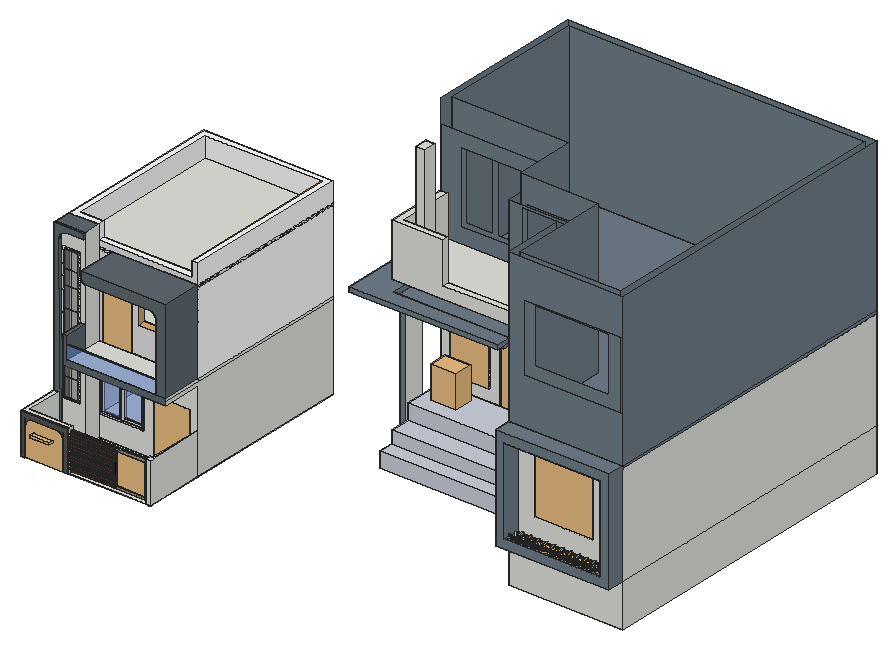
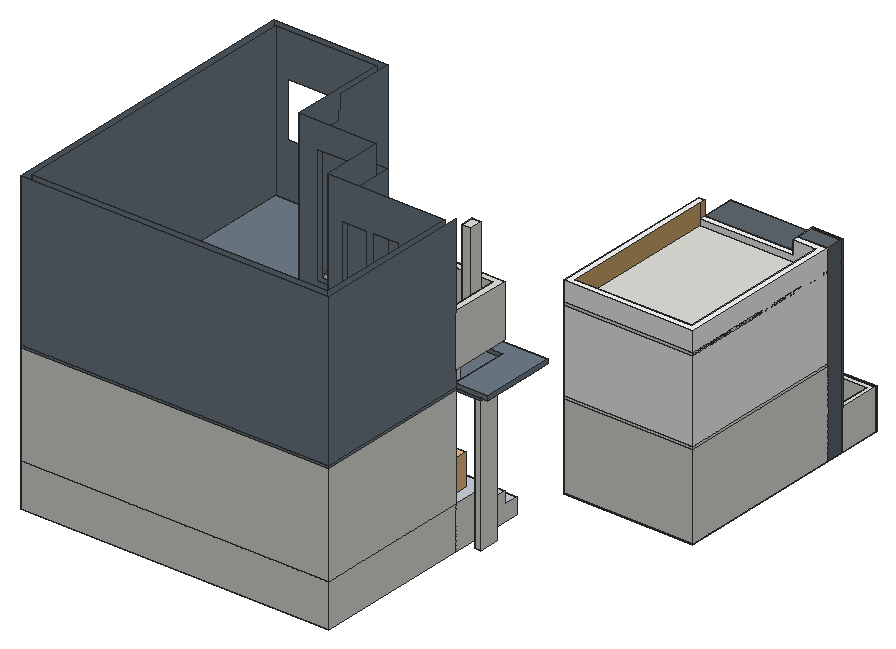
# SketchUp Ruby script. Lengths in inches.
U = 1.inch
M = Sketchup.active_model
def pt(a) = Geom::Point3d.new(a.map { |v| v * U })
def face(e, loops, mat)
  f = e.add_face(loops[0].map { |a| pt(a) })
  loops[1..].each { |l| e.add_face(l.map { |a| pt(a) }).erase! }
  f.material = f.back_material = mat if mat
  f
end
# faces: each face lists its corners as indices into pts; further lists are holes
def faces(e, pts, list, mat = nil) = list.each { |f| face(e, (f[0].is_a?(Array) ? f : [f]).map { |l| l.map { |i| pts[i] } }, mat) }
# xy, xz, yz: faces in a plane at the given z, y or x. An outline is a flat list of corners, or four numbers for a rectangle; further outlines are holes
def ring(l) = l.size == 4 ? [[l[0], l[1]], [l[2], l[1]], [l[2], l[3]], [l[0], l[3]]] : l.each_slice(2).to_a
def flat(e, list, mat, &to3) = list.each { |f| face(e, (f[0].is_a?(Array) ? f : [f]).map { |l| ring(l).map { |u, v| to3.(u, v) } }, mat) }
def xy(e, z, list, mat = nil) = flat(e, list, mat) { |x, y| [x, y, z] }
def xz(e, y, list, mat = nil) = flat(e, list, mat) { |x, z| [x, y, z] }
def yz(e, x, list, mat = nil) = flat(e, list, mat) { |y, z| [x, y, z] }
def lines(e, pts, list) = list.each { |a, b| e.add_line(pt(pts[a]), pt(pts[b])) }
# prism: a flat outline (further loops are holes) pulled along v
def prism(e, loops, v, mat = nil)
  f = face(e, loops, mat); d = Geom::Vector3d.new(v.map { |x| x * U })
  f.pushpull(f.normal.samedirection?(d) ? d.length : -d.length)
end
def box(e, o, s, mat = nil) = prism(e, [[o, [o[0] + s[0], o[1], o[2]], [o[0] + s[0], o[1] + s[1], o[2]], [o[0], o[1] + s[1], o[2]]]], [0, 0, s[2]], mat)
def at(x, y, z, deg = 0) = Geom::Transformation.translation(pt([x, y, z])) * Geom::Transformation.rotation(ORIGIN, Z_AXIS, deg.degrees)
def axes(o, x, y, z) = Geom::Transformation.new([*x, 0, *y, 0, *z, 0, *pt(o).to_a, 1])
def part(name) = M.definitions.add(name)
# library, detail: a bought-in or finely detailed component or shape, given as its bounding box
def library(name, o, s) = part(name).tap { |d| box(d.entities, o, s) }
def detail(e, o, s) = box(e.add_group.entities, o, s)
def put(e, d, t, mat = nil) = e.add_instance(d, t).tap { |i| i.material = mat if mat }
def group(e, t, mat = nil) = e.add_group.tap { |g| g.transformation = t; g.material = mat if mat }.entities
root = M.entities
M.materials.add("Aluminum_Bumpy_5cm\#1").color = [83, 85, 85]
M.materials.add("Heather_Brim").color = [96, 66, 40]
M.materials.add("Heather_Brim1").color = [73, 50, 31]
M.materials.add("Heather_Cuffs").color = [111, 126, 137]
M.materials.add("Heather_Hat").color = [155, 148, 119]
M.materials.add("Lily_Blonde").color = [204, 166, 109]
M.materials.add("Lily_Light").color = [247, 247, 197]
M.materials.add("[Color E05]").color = [255, 255, 0]
M.materials.add("[Color M01]").color = [226, 226, 226]
M.materials.add("[Color M02]").color = [198, 198, 198]
M.materials.add("[Color M09]").color = [0, 0, 0]
M.materials.add("[Formica Speckled Grey]").color = [94, 105, 111]
M.materials.add("[Marble Carrara Floor Tile]").color = [204, 208, 219]
M.materials.add("[Quartz Light Grey]").color = [251, 251, 252]
M.materials.add("[Translucent Glass Blue]").color = [100, 149, 237]
M.materials["[Translucent Glass Blue]"].alpha = 0.5
M.materials.add("[Translucent Glass Gray]").color = [128, 128, 128]
M.materials["[Translucent Glass Gray]"].alpha = 0.5
M.materials.add("[Wood Veneer 01]").color = [120, 70, 37]
c1 = library("Plant",[0,0,0],[12.59,12.59,14.16])
c2 = library("Door+01",[0,-2.84,-4],[33.31,7.1,94])
c3 = library("BANK+STOEL+MET+RONDE+LEUNING",[-13.09,-13.32,0],[26.18,25.9,25.63])
c4 = library("Group\#16",[13.45,-2,0],[53.92,2,50.83])
c5 = part("Horizontal slat")
xy(c5.entities,0,[[0,0,63.76,1]])
xy(c5.entities,1.75,[[0,0,63.76,1]],"Heather_Brim")
xz(c5.entities,0,[[0,0,63.76,1.75]],"Heather_Brim")
xz(c5.entities,1,[[0,0,63.76,1.75]])
yz(c5.entities,0,[[0,0,1,1.75]])
yz(c5.entities,63.76,[[0,0,1,1.75]])
c6 = part("Group\#20")
put(c6.entities,c5,at(0,-1,0))
c7 = library("Group\#19",[0,-1,-41.22],[40.08,1.95,42.17])
c8 = part("Difference\#2")
xy(c8.entities,0,[[0,-85,0,-27,6.6875,-27,6.6875,-77.875,63.37,-77.875,63.37,-85],[63.37,-85,67.37,-77.875],[177.37,-85,177.37,-77.875,181.37,-77.875,181.37,0,184,0,184,-85],[0,0,0,240,184,240,184,0,171.48,0,171.48,9,175,9,175,231,9,231,9,9,120.45,9,120.45,0]])
xy(c8.entities,2.75,[[131.125,-83.25,131.125,-82.25,67.37,-82.25,67.37,-80.625,177.37,-80.625,177.37,-83.25]])
xy(c8.entities,5.83,[[134.21,-83.25,174.29,-82.25]])
xy(c8.entities,29.83,[[42.47,0,105.68,9]])
xy(c8.entities,51.72,[[134.21,-83.25,174.29,-82.25]])
xy(c8.entities,54.8,[[131.125,-83.25,177.37,-83.25,177.37,-80.625,67.37,-80.625,67.37,-82.25,131.125,-82.25]])
xy(c8.entities,57.55,[[0,-85,63.37,-85,63.37,-77.875,6.6875,-77.875,6.6875,-27,0,-27],[63.37,-85,67.37,-77.875],[177.37,-85,184,-85,184,0,181.37,0,181.37,-77.875,177.37,-77.875]])
xy(c8.entities,79.83,[[42.47,0,105.68,9]])
xy(c8.entities,81,[[120.45,0,171.48,9]])
xy(c8.entities,115.1,[[36.47,-57,36.47,-24,42.47,-24,42.47,0,184,0,184,-57]],"[Formica Speckled Grey]")
xy(c8.entities,124,[[42.47,-57,168.74,0],[168.74,-57,171.48,0],[171.48,-57,184,0]])
xy(c8.entities,155,[[36.47,-57,42.47,-24]],"[Formica Speckled Grey]")
xy(c8.entities,228.74,[[69.63,-57,159.02,0]],"[Formica Speckled Grey]")
xy(c8.entities,244,[[62,-57,184,0]],"[Formica Speckled Grey]")
xz(c8.entities,-85,[[0,0,67.37,57.55],[177.37,0,184,57.55]])
xz(c8.entities,-83.25,[[[131.125,2.75,177.37,54.8],[134.21,5.83,174.29,51.72]]],"Heather_Hat")
xz(c8.entities,-82.25,[[67.37,2.75,131.125,53.05]])
xz(c8.entities,-82.25,[[134.21,5.83,174.29,48.6875],[134.21,49.64,174.29,51.72]],"Heather_Hat")
xz(c8.entities,-80.625,[[67.37,2.75,177.37,54.8]])
xz(c8.entities,-77.875,[[6.6875,0,63.37,57.55],[63.37,0,67.37,57.55],[177.37,0,181.37,57.55]])
xz(c8.entities,-57,[[36.47,115.1,184,115.1,184,124,42.47,124,42.47,155,36.47,155],[168.74,124,184,124,184,244,62,244,62,236.37,62.07,235.37,62.26,234.39,62.58,233.45,63.02,232.55,63.58,231.72,64.24,230.97,64.99,230.3125,65.82,229.76,66.71,229.32,67.66,229,68.64,228.8,69.63,228.74,159.02,228.74,160.29,228.65,161.54,228.41,162.74,228,163.88,227.4375,164.9375,226.73,165.89,225.89,166.73,224.9375,167.4375,223.88,168,222.74,168.41,221.54,168.65,220.29,168.74,219.02]],"[Formica Speckled Grey]")
xz(c8.entities,-27,[[0,0,6.6875,57.55]])
xz(c8.entities,-24,[[36.47,115.1,42.47,155]])
xz(c8.entities,0,[[0,0,42.47,120],[42.47,0,120.45,0,120.45,81,171.48,81,171.48,0,181.37,0,181.37,57.55,184,57.55,184,115.1,42.47,115.1,42.47,79.83,105.68,79.83,105.68,29.83,42.47,29.83],[181.37,0,184,57.55],[168.74,124,168.74,219.02,168.65,220.29,168.41,221.54,168,222.74,167.4375,223.88,166.73,224.9375,165.89,225.89,164.9375,226.73,163.88,227.4375,162.74,228,161.54,228.41,160.29,228.65,159.02,228.74,69.63,228.74,68.64,228.8,67.66,229,66.71,229.32,65.82,229.76,64.99,230.3125,64.24,230.97,63.58,231.72,63.02,232.55,62.58,233.45,62.26,234.39,62.07,235.37,62,236.37,62,244,184,244,184,124]])
xz(c8.entities,9,[[[9,0,9,120,175,120,175,0,171.48,0,171.48,81,120.45,81,120.45,0],[42.47,29.83,105.68,79.83]]])
xz(c8.entities,231,[[9,0,175,120]])
xz(c8.entities,240,[[0,0,184,120]])
yz(c8.entities,0,[[-85,0,-27,57.55],[0,0,240,120]])
yz(c8.entities,6.6875,[[-77.875,0,-27,57.55]])
yz(c8.entities,9,[[9,0,231,120]])
yz(c8.entities,36.47,[[-57,115.1,-24,155]],"[Formica Speckled Grey]")
yz(c8.entities,42.47,[[0,29.83,9,79.83],[-24,115.1,0,124]])
yz(c8.entities,42.47,[[-57,124,-24,155]],"[Formica Speckled Grey]")
yz(c8.entities,62,[[-57,236.37,0,244]],"[Formica Speckled Grey]")
yz(c8.entities,67.37,[[[-85,0,-77.875,57.55],[-82.25,2.75,-80.625,54.8]],[-82.25,2.75,-80.625,54.8]])
yz(c8.entities,105.68,[[0,29.83,9,79.83]])
yz(c8.entities,120.45,[[0,0,9,81]])
yz(c8.entities,131.125,[[-83.25,2.75,-82.25,53.05],[-83.25,53.05,-82.25,54.8]])
yz(c8.entities,134.21,[[-83.25,5.83,-82.25,51.72]])
yz(c8.entities,168.74,[[-57,124,0,219.02]],"[Formica Speckled Grey]")
yz(c8.entities,171.48,[[0,0,9,81]])
yz(c8.entities,174.29,[[-83.25,5.83,-82.25,51.72]])
yz(c8.entities,175,[[9,0,231,120]])
yz(c8.entities,177.37,[[[-85,0,-77.875,57.55],[-83.25,2.75,-80.625,54.8]]])
yz(c8.entities,181.37,[[-77.875,0,0,57.55]])
yz(c8.entities,184,[[-85,0,0,57.55],[0,0,240,0,240,120,-57,120,-57,115.1,0,115.1],[-57,120,0,124]])
yz(c8.entities,184,[[-57,124,0,244]],"[Formica Speckled Grey]")
p = [[168.74,-57,219.02],[168.65,-57,220.29],[168.65,0,220.29],[168.74,0,219.02],[168.41,-57,221.54],[168.41,0,221.54],
  [168,-57,222.74],[168,0,222.74],[167.4375,-57,223.88],[167.4375,0,223.88],[166.73,-57,224.9375],[166.73,0,224.9375],
  [165.89,-57,225.89],[165.89,0,225.89],[164.9375,-57,226.73],[164.9375,0,226.73],[163.88,-57,227.4375],[163.88,0,227.4375],
  [162.74,-57,228],[162.74,0,228],[161.54,-57,228.41],[161.54,0,228.41],[160.29,-57,228.65],[160.29,0,228.65],
  [69.63,-57,228.74],[68.64,-57,228.8],[68.64,0,228.8],[69.63,0,228.74],[159.02,-57,228.74],[159.02,0,228.74],
  [67.66,-57,229],[67.66,0,229],[66.71,-57,229.32],[66.71,0,229.32],[65.82,-57,229.76],[65.82,0,229.76],
  [64.99,-57,230.3125],[64.99,0,230.3125],[64.24,-57,230.97],[64.24,0,230.97],[63.58,-57,231.72],[63.58,0,231.72],
  [63.02,-57,232.55],[63.02,0,232.55],[62.58,-57,233.45],[62.58,0,233.45],[62.26,-57,234.39],[62.26,0,234.39],
  [62.07,-57,235.37],[62.07,0,235.37],[62,-57,236.37],[62,0,236.37]]
faces(c8.entities,p,[[0,1,2,3],[1,4,5,2],[4,6,7,5],[6,8,9,7],[8,10,11,9],[10,12,13,11],[12,14,15,13],[14,16,17,15],
  [16,18,19,17],[18,20,21,19],[20,22,23,21],[24,25,26,27],[22,28,29,23],[25,30,31,26],[30,32,33,31],[32,34,35,33],
  [34,36,37,35],[36,38,39,37],[38,40,41,39],[40,42,43,41],[42,44,45,43],[44,46,47,45],[46,48,49,47],[48,50,51,49]],"[Formica Speckled Grey]")
g1 = group(c8.entities,at(0,0,0))
xy(g1,0,[[0,-24,42.47,0]])
xy(g1,272,[[0,-24,42.47,0]],"[Formica Speckled Grey]")
xz(g1,-24,[[[0,0,42.47,272],[9.66,49.08,35.19,244.6]]])
xz(g1,-24,[[[11.42,50.84,33.42,242.84],[13.08,52.5,31.77,241.1875]]],"[Formica Speckled Grey]")
xz(g1,-24,[[[9.66,49.08,35.19,244.6],[11.42,50.84,33.42,242.84]]],"[Quartz Light Grey]")
xz(g1,-24,[[13.08,52.5,22.42,78.76],[22.42,52.5,31.77,78.76],[13.08,78.76,22.42,124.46],[22.42,78.76,31.77,124.46],[13.08,124.46,22.42,165.11],
  [22.42,124.46,31.77,165.11],[13.08,165.11,22.42,194.74],[22.42,165.11,31.77,194.74],[13.08,194.74,22.42,215.66],[22.42,194.74,31.77,215.66],
  [13.08,215.66,22.42,241.1875],[22.42,215.66,31.77,241.1875]],"[Translucent Glass Gray]")
xz(g1,0,[[0,0,42.47,272]])
yz(g1,0,[[-24,0,0,272]],"[Formica Speckled Grey]")
yz(g1,42.47,[[-24,0,0,272]])
g2 = group(g1,at(0,-27,0))
prism(g2,[[[16.68,0,263.77],[18.12,0,263.86],[42.47,0,263.86],[42.47,0,272],[0,0,272],[0,0,0],[9.08,0,0],[7.08,0,252.82],[7.17,0,254.26],[7.45,0,255.68],[7.92,0,257.04],[8.56,0,258.34],[9.36,0,259.54],[10.3125,0,260.625],[11.4,0,261.58],[12.6,0,262.38],[13.89,0,263.02],[15.26,0,263.49]]],[0,3,0],"[Formica Speckled Grey]")
g3 = group(c8.entities,at(257.96,-85,32.54),"Aluminum_Bumpy_5cm\#1")
g4 = group(g3,at(-257.96,-2,-32.54))
prism(g4,[[[60.56,0,41.6],[60.65,0,40.21],[60.65,0,0],[63.37,0,0],[67.37,0,0],[67.37,0,57.55],[63.37,0,57.55],[0,0,57.55],[0,0,0],[6.72,0,0],[6.72,0,39.6],[6.82,0,41.0625],[7.11,0,42.5],[7.58,0,43.9],[8.23,0,45.21],[9.04,0,46.43],[10.01,0,47.54],[11.12,0,48.51],[12.34,0,49.32],[13.66,0,49.97],[15.05,0,50.45],[16.49,0,50.73],[17.95,0,50.83],[50.03,0,50.83],[51.42,0,50.74],[52.78,0,50.47],[54.09,0,50.02],[55.34,0,49.41],[56.49,0,48.63],[57.54,0,47.72],[58.45,0,46.68],[59.22,0,45.52],[59.84,0,44.28],[60.28,0,42.96]]],[0,2,0])
p = [[60.65,2,0],[6.72,2,0]]
lines(g4,p,[[0,1]])
put(c8.entities,c4,at(-7.16,-84.84,0),"Heather_Brim1")
g5 = group(c8.entities,at(67.37,-82.25,53.05))
put(g5,c5,at(0,-1,0))
put(c8.entities,c6,at(67.37,-82.25,51.04))
put(c8.entities,c6,at(67.37,-82.25,49.03))
put(c8.entities,c6,at(67.37,-82.25,47.01))
put(c8.entities,c6,at(67.37,-82.25,45))
put(c8.entities,c6,at(67.37,-82.25,42.99))
put(c8.entities,c6,at(67.37,-82.25,40.98))
put(c8.entities,c6,at(67.37,-82.25,38.97))
put(c8.entities,c6,at(67.37,-82.25,36.95))
put(c8.entities,c6,at(67.37,-82.25,34.94))
put(c8.entities,c6,at(67.37,-82.25,32.93))
put(c8.entities,c6,at(67.37,-82.25,30.92))
put(c8.entities,c6,at(67.37,-82.25,28.91))
put(c8.entities,c6,at(67.37,-82.25,26.89))
put(c8.entities,c6,at(67.37,-82.25,24.88))
put(c8.entities,c6,at(67.37,-82.25,22.87))
put(c8.entities,c6,at(67.37,-82.25,20.86))
put(c8.entities,c6,at(67.37,-82.25,18.85))
put(c8.entities,c6,at(67.37,-82.25,16.83))
put(c8.entities,c6,at(67.37,-82.25,14.82))
put(c8.entities,c6,at(67.37,-82.25,12.81))
put(c8.entities,c6,at(67.37,-82.25,10.8))
put(c8.entities,c6,at(67.37,-82.25,8.79))
put(c8.entities,c6,at(67.37,-82.25,6.77))
put(c8.entities,c6,at(67.37,-82.25,4.76))
put(c8.entities,c6,at(67.37,-82.25,2.75))
put(c8.entities,c7,at(134.21,-82.25,48.6875))
c9 = library("modern+double+door",[0,0,0],[3.2,48,90])
c10 = part("Difference")
xy(c10.entities,0,[[278,0,278,139,167,139,167,226,155.98,226,155.98,235,176,235,176,148,287,148,287,9,431,9,431,443,9,443,9,235,85.04,235,85.04,226,0,226,0,452,440,452,440,0]])
xy(c10.entities,17.15,[[14.41,226,69.41,235]])
xy(c10.entities,39,[[315.41,0,397.84,9]])
xy(c10.entities,122.51,[[85.04,226,155.98,235]])
xy(c10.entities,125,[[315.41,0,397.84,9]])
xy(c10.entities,130.15,[[14.41,226,69.41,235]])
xy(c10.entities,144,[[[278,0,440,0,440,452,0,452,0,226,167,226,167,139,278,139],[287,9,287,148,176,148,176,235,9,235,9,443,431,443,431,9]]])
xz(c10.entities,0,[[[278,0,440,144],[315.41,39,397.84,125]]])
xz(c10.entities,9,[[[287,0,431,144],[315.41,39,397.84,125]]])
xz(c10.entities,139,[[167,0,278,144]])
xz(c10.entities,148,[[176,0,287,144]])
xz(c10.entities,226,[[[0,0,85.04,0,85.04,122.51,155.98,122.51,155.98,0,167,0,167,144,0,144],[14.41,17.15,69.41,130.15]],[0,144,167,148]])
xz(c10.entities,235,[[[9,0,9,144,176,144,176,0,155.98,0,155.98,122.51,85.04,122.51,85.04,0],[14.41,17.15,69.41,130.15]]])
xz(c10.entities,443,[[9,0,431,144]])
xz(c10.entities,452,[[0,0,440,144]])
yz(c10.entities,0,[[226,0,452,144]])
yz(c10.entities,9,[[235,0,443,144]])
yz(c10.entities,14.41,[[226,17.15,235,130.15]])
yz(c10.entities,69.41,[[226,17.15,235,130.15]])
yz(c10.entities,85.04,[[226,0,235,122.51]])
yz(c10.entities,155.98,[[226,0,235,122.51]])
yz(c10.entities,167,[[139,0,226,144]])
yz(c10.entities,176,[[148,0,235,144]])
yz(c10.entities,278,[[0,0,139,144]])
yz(c10.entities,287,[[9,0,148,144]])
yz(c10.entities,315.41,[[0,39,9,125]])
yz(c10.entities,397.84,[[0,39,9,125]])
yz(c10.entities,431,[[9,0,443,144]])
yz(c10.entities,440,[[0,0,452,144]])
c11 = part("Group\#65")
detail(c11.entities,[0,0,0],[5.71,82.68,6.45])
c12 = part("Group\#68")
put(c12.entities,c11,axes([28.08,0,71.6],[1,0,0],[0,0.5,-0.86603],[0,0.86603,0.5]))
put(c12.entities,c11,axes([2.85,59.63,58],[-0.405,-0.70148,0],[0.35074,-0.2025,-0.70148],[0.6075,-0.35074,0.405]))
put(c12.entities,c11,axes([-1.6,23.09,64.44],[0.55484,-0.83195,0],[0.37438,0.24968,-0.77942],[0.72049,0.48051,0.5]))
c13 = part("Group\#69")
put(c13.entities,c11,axes([28.08,0,71.6],[1,0,0],[0,0.5,-0.86603],[0,0.86603,0.5]))
put(c13.entities,c11,axes([2.85,59.63,58],[-0.405,-0.70148,0],[0.35074,-0.2025,-0.70148],[0.6075,-0.35074,0.405]))
put(c13.entities,c11,axes([-1.6,23.09,64.44],[0.55484,-0.83195,0],[0.37438,0.24968,-0.77942],[0.72049,0.48051,0.5]))
c14 = part("Group\#75")
put(c14.entities,c12,at(0.8125,72.29,3.66,-90))
put(c14.entities,c13,at(11.2,0,3.66))
put(c14.entities,c13,axes([83.03,10.65,3.66],[0,1,0],[-1,0,0],[0,0,0.6674]))
put(c14.entities,c12,axes([10.73,0.27,3.66],[1,0,0],[0,1,0],[0,0,0.6674]))
put(c14.entities,c12,axes([0,74.01,0],[0,-1,0],[1,0,0],[0,0,0.6674]))
put(c14.entities,c13,axes([10.39,1.72,0],[1,0,0],[0,1,0],[0,0,0.6674]))
c15 = library("okno",[0,0,0],[1.97,20.83,48.43])
c16 = part("Group\#8")
xy(c16.entities,0,[[0,0,19.69,39.37]])
c17 = part("Group\#9")
prism(c17.entities,[[[45.28,43.31,0],[45.28,0,0],[21.65,0,0],[21.65,43.31,0]],[[23.62,41.34,0],[23.62,1.97,0],[43.31,1.97,0],[43.31,41.34,0]]],[0,0,1.97])
c18 = part("Group\#13")
g6 = group(c18.entities,at(1.97,1.97,0))
put(g6,c16,at(1.97,1.97,0.98),"[Translucent Glass Blue]")
put(g6,c17,at(-21.65,0,0))
g7 = group(c18.entities,at(23.62,1.97,1.97))
put(g7,c16,at(1.97,1.97,0.98),"[Translucent Glass Blue]")
put(g7,c17,at(-21.65,0,0))
g8 = group(c18.entities,at(0,0,3.9375))
prism(g8,[[[0,47.24,-3.9375],[49.21,47.24,-3.9375],[49.21,0,-3.9375],[0,0,-3.9375]],[[1.97,1.97,-3.9375],[47.24,1.97,-3.9375],[47.24,45.28,-3.9375],[1.97,45.28,-3.9375]]],[0,0,3.9375])
c19 = library("HOUSE 301",[0.15,0,0],[27.16,3.125,6])
c20 = library("normal+window",[0,0,0],[4.84,65.35,84.65])
c21 = part("Difference\#1")
xy(c21.entities,0,[[0,0,0,240,184,240,184,0,171.48,0,171.48,9,175,9,175,231,9,231,9,9,47.47,9,47.47,0],[47.47,0,88.68,9],[88.68,0,171.48,9]],"Lily_Blonde")
xy(c21.entities,79.83,[[47.47,0,88.68,9]],"Lily_Blonde")
xy(c21.entities,81,[[99.45,0,157.48,9]],"Lily_Blonde")
xy(c21.entities,128,[[42.47,0,175,9]],"[Quartz Light Grey]")
xy(c21.entities,148,[[0,0,42.47,0,42.47,9,9,9,9,231,175,231,175,0,184,0,184,240,0,240]],"[Quartz Light Grey]")
xz(c21.entities,0,[[[42.47,0,47.47,0,47.47,79.83,88.68,79.83,88.68,0,184,0,184,148,175,148,175,128,42.47,128],[99.45,38.13,157.48,81]]],"[Color M01]")
xz(c21.entities,9,[[[9,0,9,148,42.47,148,42.47,128,175,128,175,0,88.68,0,88.68,79.83,47.47,79.83,47.47,0],[99.45,40.5,157.48,81]]],"[Quartz Light Grey]")
xz(c21.entities,231,[[9,0,175,148]],"[Quartz Light Grey]")
xz(c21.entities,240,[[0,0,184,148]],"[Quartz Light Grey]")
yz(c21.entities,0,[[0,0,240,148]],"[Quartz Light Grey]")
yz(c21.entities,9,[[9,0,231,148]],"[Quartz Light Grey]")
yz(c21.entities,42.47,[[0,128,9,148]],"[Quartz Light Grey]")
yz(c21.entities,47.47,[[0,0,9,79.83]],"Lily_Blonde")
yz(c21.entities,88.68,[[0,0,9,79.83]],"Lily_Blonde")
yz(c21.entities,99.45,[[0,38.13,9,40.5,9,81,0,81]],"Lily_Blonde")
yz(c21.entities,157.48,[[0,38.13,0,81,9,81,9,40.5]],"Lily_Blonde")
yz(c21.entities,175,[[9,0,231,148],[0,128,9,148]],"Lily_Blonde")
yz(c21.entities,184,[[0,0,240,148]],"[Quartz Light Grey]")
p = [[99.45,9,40.5],[99.45,0,38.13],[157.48,0,38.13],[157.48,9,40.5]]
faces(c21.entities,p,[[0,1,2,3]],"Lily_Blonde")
c22 = library("door by lz",[5.91,-4.92,0],[35.43,6.61,78.74])
box(root,[0,2,-1],[184,325,1])
xy(root,-61,[[540.22,194.96,540.22,333.96,429.22,333.96,429.22,420.96,262.22,420.96,262.22,646.96,702.22,646.96,702.22,194.96],[262.22,312.18,429.22,420.96],[242.22,372.96,251.22,400.96]])
xy(root,-39,[[262.22,312.18,429.22,333.18]],"[Marble Carrara Floor Tile]")
xy(root,-22,[[262.22,333.18,429.22,362.96]],"[Marble Carrara Floor Tile]")
xy(root,0,[[540.22,194.96,702.22,194.96,702.22,646.96,262.22,646.96,262.22,420.96,429.22,420.96,429.22,333.96,540.22,333.96]])
xy(root,0,[[262.22,362.96,429.22,420.96]],"[Marble Carrara Floor Tile]")
xy(root,22.04,[[131.8,0.75,133.8,3.75]],"[Color M09]")
xy(root,37.04,[[131.8,0.75,133.8,3.75]],"[Color M09]")
xy(root,134.48,[[581.55,179.5625,581.04,179.63,580.55,179.83,580.14,180.15,579.82,180.5625,579.62,181.04,579.55,181.5625,579.62,182.08,579.82,182.5625,580.14,182.98,580.55,183.29,581.04,183.49,581.55,183.5625,582.07,183.49,582.55,183.29,582.97,182.98,583.29,182.5625,583.49,182.08,583.55,181.5625,583.49,181.04,583.29,180.5625,582.97,180.15,582.55,179.83,582.07,179.63],[625.07,179.5625,624.55,179.63,624.07,179.83,623.65,180.15,623.34,180.5625,623.14,181.04,623.07,181.5625,623.14,182.08,623.34,182.5625,623.65,182.98,624.07,183.29,624.55,183.49,625.07,183.5625,625.59,183.49,626.07,183.29,626.48,182.98,626.8,182.5625,627,182.08,627.07,181.5625,627,181.04,626.8,180.5625,626.48,180.15,626.07,179.83,625.59,179.63],[669.07,179.5625,668.55,179.63,668.07,179.83,667.65,180.15,667.34,180.5625,667.14,181.04,667.07,181.5625,667.14,182.08,667.34,182.5625,667.65,182.98,668.07,183.29,668.55,183.49,669.07,183.5625,669.59,183.49,670.07,183.29,670.48,182.98,670.8,182.5625,671,182.08,671.07,181.5625,671,181.04,670.8,180.5625,670.48,180.15,670.07,179.83,669.59,179.63]],"[Color E05]")
xy(root,135.48,[[581.55,179.5625,582.07,179.63,582.55,179.83,582.97,180.15,583.29,180.5625,583.49,181.04,583.55,181.5625,583.49,182.08,583.29,182.5625,582.97,182.98,582.55,183.29,582.07,183.49,581.55,183.5625,581.04,183.49,580.55,183.29,580.14,182.98,579.82,182.5625,579.62,182.08,579.55,181.5625,579.62,181.04,579.82,180.5625,580.14,180.15,580.55,179.83,581.04,179.63],[625.07,179.5625,625.59,179.63,626.07,179.83,626.48,180.15,626.8,180.5625,627,181.04,627.07,181.5625,627,182.08,626.8,182.5625,626.48,182.98,626.07,183.29,625.59,183.49,625.07,183.5625,624.55,183.49,624.07,183.29,623.65,182.98,623.34,182.5625,623.14,182.08,623.07,181.5625,623.14,181.04,623.34,180.5625,623.65,180.15,624.07,179.83,624.55,179.63],[669.07,179.5625,669.59,179.63,670.07,179.83,670.48,180.15,670.8,180.5625,671,181.04,671.07,181.5625,671,182.08,670.8,182.5625,670.48,182.98,670.07,183.29,669.59,183.49,669.07,183.5625,668.55,183.49,668.07,183.29,667.65,182.98,667.34,182.5625,667.14,182.08,667.07,181.5625,667.14,181.04,667.34,180.5625,667.65,180.15,668.07,179.83,668.55,179.63]])
xy(root,143,[[42.47,30,168.47,31]],"[Wood Veneer 01]")
xy(root,144,[[242.22,372.96,251.22,400.96]])
xy(root,144,[[42.47,30,168.47,31]],"[Wood Veneer 01]")
xy(root,148,[[272.22,401.96,429.22,420.96]])
xy(root,148,[[[540.22,194.96,540.22,333.96,429.22,333.96,429.22,420.96,262.22,420.96,262.22,646.96,702.22,646.96,702.22,194.96],[549.22,203.96,693.22,203.96,693.22,637.96,271.22,637.96,271.22,429.96,438.22,429.96,438.22,342.96,549.22,342.96]]],"Heather_Cuffs")
xy(root,170.89,[[262.22,333.96,272.22,420.96],[272.22,333.96,429.22,401.96],[272.22,401.96,429.22,420.96]])
xy(root,188.26,[[335.26,333.96,429.22,342.96],[[272.2,342.96,429.22,420.96],[272.78,362.97,285.78,380.97]]])
xy(root,245.97,[[262.22,333.96,335.26,333.96,335.26,342.96,272.2,342.96,272.2,420.96,262.22,420.96]])
xy(root,331,[[272.78,362.97,285.78,380.97]])
xz(root,0.75,[[131.8,22.04,133.8,37.04]],"[Color M09]")
xz(root,3.75,[[131.8,22.04,133.8,37.04]])
xz(root,30,[[42.47,124,168.74,143]],"[Translucent Glass Blue]")
xz(root,30,[[42.47,143,168.47,144]],"[Wood Veneer 01]")
xz(root,31,[[42.47,143,168.47,144]],"[Wood Veneer 01]")
xz(root,194.96,[[540.22,-61,702.22,0]])
xz(root,194.96,[[540.22,148,702.22,148,702.22,214.89,561.22,214.89,561.22,310.89,702.22,310.89,702.22,363.8,540.22,363.8]],"Heather_Cuffs")
xz(root,203.96,[[[549.22,148,693.22,363.8],[569.63,225,675.0625,303]]],"Heather_Cuffs")
xz(root,312.18,[[262.22,-61,429.22,-39]],"[Marble Carrara Floor Tile]")
xz(root,333.18,[[262.22,-39,429.22,-22]],"[Marble Carrara Floor Tile]")
xz(root,333.96,[[429.22,-61,540.22,0],[262.22,170.89,429.22,170.89,429.22,188.26,335.26,188.26,335.26,245.97,262.22,245.97]])
xz(root,333.96,[[[429.22,148,540.22,331],[447.88,158.93,522.88,327.93]]],"Heather_Cuffs")
xz(root,342.96,[[272.2,188.26,335.26,245.97]])
xz(root,342.96,[[[438.22,148,549.22,363.8],[447.88,158.93,522.88,327.93]]],"Heather_Cuffs")
xz(root,362.96,[[262.22,-22,429.22,0]],"[Marble Carrara Floor Tile]")
xz(root,362.97,[[272.78,188.26,285.78,331]])
xz(root,372.96,[[242.22,-61,251.22,144]],"Heather_Cuffs")
xz(root,380.97,[[272.78,188.26,285.78,331]])
xz(root,400.96,[[242.22,-61,251.22,144]])
xz(root,401.96,[[272.22,148,429.22,170.89]])
xz(root,420.96,[[262.22,-61,429.22,0],[272.22,148,429.22,170.89],[262.22,188.26,272.2,245.97]])
xz(root,420.96,[[[262.22,148,429.22,331],[290.7,209.8,417.7,310.8]]],"Heather_Cuffs")
xz(root,429.96,[[[271.22,148,438.22,363.8],[290.7,209.8,329.6,310.8],[336.74,209.8,373.65,310.8],[381.73,209.8,417.7,310.8]]],"Heather_Cuffs")
xz(root,637.96,[[271.22,148,693.22,363.8]],"Heather_Cuffs")
xz(root,646.96,[[262.22,-61,702.22,0]])
xz(root,646.96,[[262.22,148,702.22,363.8]],"Heather_Cuffs")
yz(root,42.47,[[30,143,31,144]],"[Wood Veneer 01]")
yz(root,131.8,[[0.75,22.04,3.75,37.04]],"[Color M09]")
yz(root,133.8,[[0.75,22.04,3.75,37.04]],"[Color M09]")
yz(root,168.47,[[30,143,31,144]],"[Wood Veneer 01]")
yz(root,242.22,[[372.96,-61,400.96,144]])
yz(root,251.22,[[372.96,-61,400.96,144]])
yz(root,262.22,[[312.18,-61,312.18,-39,333.18,-39,333.18,-22,362.96,-22,362.96,0,420.96,0,420.96,-61],[420.96,-61,646.96,0],[333.96,170.89,420.96,245.97]])
yz(root,262.22,[[420.96,148,646.96,363.8]],"Heather_Cuffs")
yz(root,271.22,[[429.96,148,637.96,363.8]],"Heather_Cuffs")
yz(root,272.2,[[342.96,188.26,420.96,245.97]])
yz(root,272.22,[[401.96,148,420.96,170.89]])
yz(root,272.78,[[362.97,188.26,380.97,331]])
yz(root,285.78,[[362.97,188.26,380.97,331]])
yz(root,335.26,[[333.96,188.26,342.96,245.97]])
yz(root,429.22,[[312.18,-61,333.96,-61,333.96,-22,333.18,-22,333.18,-39,312.18,-39],[333.96,-61,420.96,-61,420.96,0,362.96,0,362.96,-22,333.96,-22],[333.96,-22,362.96,0],[401.96,148,420.96,170.89],[333.96,170.89,420.96,188.26]])
yz(root,429.22,[[333.96,148,420.96,331]],"Heather_Cuffs")
yz(root,438.22,[[342.96,148,429.96,363.8]],"Heather_Cuffs")
yz(root,540.22,[[194.96,-61,333.96,0]])
yz(root,540.22,[[194.96,148,194.96,363.8,278.96,363.8,278.96,343,281.96,343,281.96,331,333.96,331,333.96,148]],"Heather_Cuffs")
yz(root,549.22,[[203.96,148,342.96,363.8]],"Heather_Cuffs")
yz(root,693.22,[[203.96,148,637.96,363.8]],"Heather_Cuffs")
yz(root,702.22,[[194.96,-61,646.96,0]])
yz(root,702.22,[[194.96,148,646.96,363.8]],"Heather_Cuffs")
p = [[581.04,179.63,135.48],[580.55,179.83,135.48],[580.55,179.83,134.48],[581.04,179.63,134.48],[581.55,179.5625,135.48],[581.55,179.5625,134.48],
  [582.07,179.63,135.48],[582.07,179.63,134.48],[582.55,179.83,135.48],[582.55,179.83,134.48],[624.55,179.63,135.48],[624.07,179.83,135.48],
  [624.07,179.83,134.48],[624.55,179.63,134.48],[625.07,179.5625,135.48],[625.07,179.5625,134.48],[625.59,179.63,135.48],[625.59,179.63,134.48],
  [626.07,179.83,135.48],[626.07,179.83,134.48],[668.55,179.63,135.48],[668.07,179.83,135.48],[668.07,179.83,134.48],[668.55,179.63,134.48],
  [669.07,179.5625,135.48],[669.07,179.5625,134.48],[669.59,179.63,135.48],[669.59,179.63,134.48],[670.07,179.83,135.48],[670.07,179.83,134.48],
  [580.14,180.15,135.48],[580.14,180.15,134.48],[582.97,180.15,135.48],[582.97,180.15,134.48],[623.65,180.15,135.48],[623.65,180.15,134.48],
  [626.48,180.15,135.48],[626.48,180.15,134.48],[667.65,180.15,135.48],[667.65,180.15,134.48],[670.48,180.15,135.48],[670.48,180.15,134.48],
  [579.82,180.5625,135.48],[579.82,180.5625,134.48],[583.29,180.5625,135.48],[583.29,180.5625,134.48],[623.34,180.5625,135.48],[623.34,180.5625,134.48],
  [626.8,180.5625,135.48],[626.8,180.5625,134.48],[667.34,180.5625,135.48],[667.34,180.5625,134.48],[670.8,180.5625,135.48],[670.8,180.5625,134.48],
  [579.62,181.04,135.48],[579.62,181.04,134.48],[583.49,181.04,135.48],[583.49,181.04,134.48],[623.14,181.04,135.48],[623.14,181.04,134.48],
  [627,181.04,135.48],[627,181.04,134.48],[667.14,181.04,135.48],[667.14,181.04,134.48],[671,181.04,135.48],[671,181.04,134.48],
  [579.55,181.5625,135.48],[579.55,181.5625,134.48],[583.55,181.5625,135.48],[583.55,181.5625,134.48],[623.07,181.5625,135.48],[623.07,181.5625,134.48],
  [627.07,181.5625,135.48],[627.07,181.5625,134.48],[667.07,181.5625,135.48],[667.07,181.5625,134.48],[671.07,181.5625,135.48],[671.07,181.5625,134.48],
  [579.62,182.08,135.48],[579.62,182.08,134.48],[583.49,182.08,135.48],[583.49,182.08,134.48],[623.14,182.08,135.48],[623.14,182.08,134.48],
  [627,182.08,135.48],[627,182.08,134.48],[667.14,182.08,135.48],[667.14,182.08,134.48],[671,182.08,135.48],[671,182.08,134.48],
  [579.82,182.5625,135.48],[579.82,182.5625,134.48],[583.29,182.5625,135.48],[583.29,182.5625,134.48],[623.34,182.5625,135.48],[623.34,182.5625,134.48],
  [626.8,182.5625,135.48],[626.8,182.5625,134.48],[667.34,182.5625,135.48],[667.34,182.5625,134.48],[670.8,182.5625,135.48],[670.8,182.5625,134.48],
  [580.14,182.98,135.48],[580.14,182.98,134.48],[582.97,182.98,135.48],[582.97,182.98,134.48],[623.65,182.98,135.48],[623.65,182.98,134.48],
  [626.48,182.98,135.48],[626.48,182.98,134.48],[667.65,182.98,135.48],[667.65,182.98,134.48],[670.48,182.98,135.48],[670.48,182.98,134.48],
  [580.55,183.29,135.48],[580.55,183.29,134.48],[582.55,183.29,135.48],[582.55,183.29,134.48],[624.07,183.29,135.48],[624.07,183.29,134.48],
  [626.07,183.29,135.48],[626.07,183.29,134.48],[668.07,183.29,135.48],[668.07,183.29,134.48],[670.07,183.29,135.48],[670.07,183.29,134.48],
  [581.04,183.49,135.48],[581.04,183.49,134.48],[582.07,183.49,135.48],[582.07,183.49,134.48],[624.55,183.49,135.48],[624.55,183.49,134.48],
  [625.59,183.49,135.48],[625.59,183.49,134.48],[668.55,183.49,135.48],[668.55,183.49,134.48],[669.59,183.49,135.48],[669.59,183.49,134.48],
  [581.55,183.5625,135.48],[581.55,183.5625,134.48],[625.07,183.5625,135.48],[625.07,183.5625,134.48],[669.07,183.5625,135.48],[669.07,183.5625,134.48]]
faces(root,p,[[0,1,2,3],[4,0,3,5],[6,4,5,7],[8,6,7,9],[10,11,12,13],[14,10,13,15],[16,14,15,17],[18,16,17,19],
  [20,21,22,23],[24,20,23,25],[26,24,25,27],[28,26,27,29],[1,30,31,2],[32,8,9,33],[11,34,35,12],[36,18,19,37],
  [21,38,39,22],[40,28,29,41],[30,42,43,31],[44,32,33,45],[34,46,47,35],[48,36,37,49],[38,50,51,39],[52,40,41,53],
  [42,54,55,43],[56,44,45,57],[46,58,59,47],[60,48,49,61],[50,62,63,51],[64,52,53,65],[54,66,67,55],[68,56,57,69],
  [58,70,71,59],[72,60,61,73],[62,74,75,63],[76,64,65,77],[66,78,79,67],[80,68,69,81],[70,82,83,71],[84,72,73,85],
  [74,86,87,75],[88,76,77,89],[78,90,91,79],[92,80,81,93],[82,94,95,83],[96,84,85,97],[86,98,99,87],[100,88,89,101],
  [90,102,103,91],[104,92,93,105],[94,106,107,95],[108,96,97,109],[98,110,111,99],[112,100,101,113],[102,114,115,103],[116,104,105,117],
  [106,118,119,107],[120,108,109,121],[110,122,123,111],[124,112,113,125],[114,126,127,115],[128,116,117,129],[118,130,131,119],[132,120,121,133],
  [122,134,135,123],[136,124,125,137],[126,138,139,127],[138,128,129,139],[130,140,141,131],[140,132,133,141],[134,142,143,135],[142,136,137,143]])
put(root,c1,axes([462.45,309.24,-61.95],[2.1504,0,0],[0,2,0],[0,0,2]))
put(root,c2,axes([120.45,88.7,-0.38],[1.53213,0,0],[0,0.59962,0],[0,0,0.90426]))
put(root,c3,axes([295.35,396.87,-0.04],[1.38816,0,0],[0,-1,0],[0,0,1.77]))
put(root,c8,at(0,87,0))
put(root,c9,axes([346.76,423.46,0],[0,-0.78125,0],[1.48834,0,0],[0,0,1.36121]))
put(root,c10,at(262.22,194.96,0))
g9 = group(root,at(540.22,194.96,0))
prism(g9,[[[162,0,0],[0,0,0],[0,0,148],[162,0,148]],[[12.52,0,135.48],[12.52,0,12.52],[149.48,0,12.52],[149.48,0,135.48]]],[0,-24,0],"Heather_Cuffs")
put(root,c14,axes([577.56,184.53,12.52],[-0.0659,-0.24592,0],[-0.24592,0.0659,0],[0,0,0.08614]))
put(root,c14,axes([589.03,184.53,12.52],[-0.0659,-0.24592,0],[-0.24592,0.0659,0],[0,0,0.08614]))
put(root,c14,axes([600.5,184.53,12.52],[-0.0659,-0.24592,0],[-0.24592,0.0659,0],[0,0,0.08614]))
put(root,c14,axes([611.97,184.53,12.52],[-0.0659,-0.24592,0],[-0.24592,0.0659,0],[0,0,0.08614]))
put(root,c14,axes([623.44,184.53,12.52],[-0.0659,-0.24592,0],[-0.24592,0.0659,0],[0,0,0.08614]))
put(root,c14,axes([634.91,184.53,12.52],[-0.0659,-0.24592,0],[-0.24592,0.0659,0],[0,0,0.08614]))
put(root,c14,axes([646.38,184.53,12.52],[-0.0659,-0.24592,0],[-0.24592,0.0659,0],[0,0,0.08614]))
put(root,c14,axes([657.86,184.53,12.52],[-0.0659,-0.24592,0],[-0.24592,0.0659,0],[0,0,0.08614]))
put(root,c14,axes([669.33,184.53,12.52],[-0.0659,-0.24592,0],[-0.24592,0.0659,0],[0,0,0.08614]))
put(root,c14,axes([680.8,184.53,12.52],[-0.0659,-0.24592,0],[-0.24592,0.0659,0],[0,0,0.08614]))
put(root,c14,axes([692.27,184.53,12.52],[-0.0659,-0.24592,0],[-0.24592,0.0659,0],[0,0,0.08614]))
put(root,c15,axes([331.63,419.64,17.15],[0,2.899,0],[-2.64006,0,0],[0,0,2.3335]))
put(root,c18,axes([42.47,87,79.83],[1.28,0,0],[0,0,-1.05833],[0,1.56718,0]))
put(root,c19,axes([18.63,0.16,32.12],[1,0,0],[0,0,1],[0,-1,0]),"Lily_Light")
put(root,c20,axes([660.0625,194.96,39],[0,1,0],[-1.26126,0,0],[0,0,1.016]))
g10 = group(root,at(0,87,120))
g11 = group(g10,at(0,0,-4.9))
xy(g11,4.9,[[0,0,184,240]])
xy(g11,8.9,[[0,0,184,240]])
xz(g11,0,[[42.47,0,184,4.9],[0,4.9,42.47,8.9],[42.47,4.9,184,8.9]])
xz(g11,240,[[0,4.9,184,8.9]])
yz(g11,0,[[0,4.9,240,8.9]])
yz(g11,184,[[0,4.9,240,8.9]])
g12 = group(g10,at(0,0,115.1))
box(g12,[0,0,4.9],[184,240,4])
put(root,c21,at(0,87,124),"[Color M02]")
put(root,c22,axes([40.59,91.1875,124],[1.16305,0,0],[0,0.85119,0],[0,0,1.01386]))
g13 = group(root,at(262.22,194.96,144),"Heather_Cuffs")
xy(g13,0,[[278,0,278,139,167,139,167,130,-36,130,-36,226,0,226,0,452,440,452,440,0]])
xy(g13,4,[[278,0,440,0,440,452,0,452,0,226,1.96,226,1.96,140.7,167,140.7,167,139,278,139],[-45,119,-20,130],[-20,119,-3,130],[-3,119,1.96,130],[1.96,119,167,130],
  [-45,130,-36,226],[-36,130,1.96,226],[1.96,130,167,140.7]])
xy(g13,10,[[-45,119,167,119,167,140.7,1.96,140.7,1.96,226,-45,226]])
xz(g13,0,[[278,0,440,4]])
xz(g13,119,[[-45,4,167,10]])
xz(g13,130,[[-36,0,167,4]])
xz(g13,139,[[167,0,278,4]])
xz(g13,140.7,[[1.96,4,167,10]])
xz(g13,226,[[-36,0,0,4],[-45,4,1.96,10]])
xz(g13,452,[[0,0,440,4]])
yz(g13,-45,[[119,4,226,10]])
yz(g13,-36,[[130,0,226,4]])
yz(g13,0,[[226,0,452,4]])
yz(g13,1.96,[[140.7,4,226,10]])
yz(g13,167,[[130,0,139,4],[119,4,140.7,10]])
yz(g13,278,[[0,0,139,4]])
yz(g13,440,[[0,0,452,4]])
